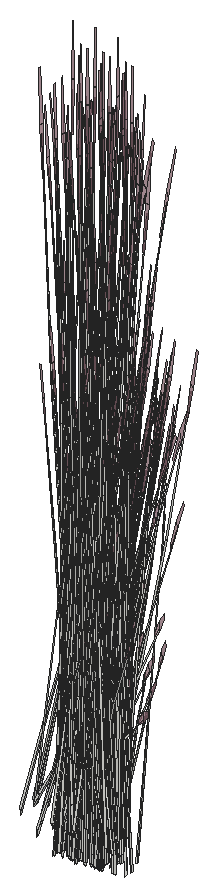
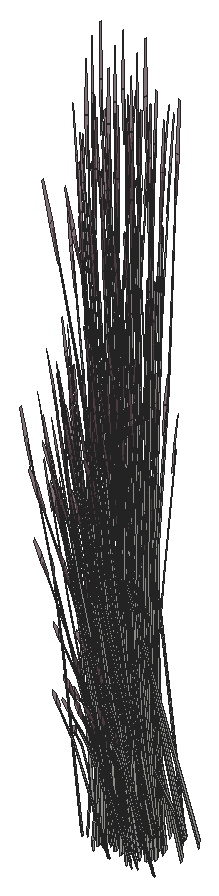
# SketchUp Ruby script. Lengths in inches.
U = 1.inch
M = Sketchup.active_model
def pt(a) = Geom::Point3d.new(a.map { |v| v * U })
def face(e, loops, mat)
  f = e.add_face(loops[0].map { |a| pt(a) })
  loops[1..].each { |l| e.add_face(l.map { |a| pt(a) }).erase! }
  f.material = f.back_material = mat if mat
  f
end
# faces: each face lists its corners as indices into pts; further lists are holes
def faces(e, pts, list, mat = nil) = list.each { |f| face(e, (f[0].is_a?(Array) ? f : [f]).map { |l| l.map { |i| pts[i] } }, mat) }
# xy, xz, yz: faces in a plane at the given z, y or x. An outline is a flat list of corners, or four numbers for a rectangle; further outlines are holes
def ring(l) = l.size == 4 ? [[l[0], l[1]], [l[2], l[1]], [l[2], l[3]], [l[0], l[3]]] : l.each_slice(2).to_a
def flat(e, list, mat, &to3) = list.each { |f| face(e, (f[0].is_a?(Array) ? f : [f]).map { |l| ring(l).map { |u, v| to3.(u, v) } }, mat) }
def xy(e, z, list, mat = nil) = flat(e, list, mat) { |x, y| [x, y, z] }
def xz(e, y, list, mat = nil) = flat(e, list, mat) { |x, z| [x, y, z] }
def yz(e, x, list, mat = nil) = flat(e, list, mat) { |y, z| [x, y, z] }
def lines(e, pts, list) = list.each { |a, b| e.add_line(pt(pts[a]), pt(pts[b])) }
# prism: a flat outline (further loops are holes) pulled along v
def prism(e, loops, v, mat = nil)
  f = face(e, loops, mat); d = Geom::Vector3d.new(v.map { |x| x * U })
  f.pushpull(f.normal.samedirection?(d) ? d.length : -d.length)
end
def box(e, o, s, mat = nil) = prism(e, [[o, [o[0] + s[0], o[1], o[2]], [o[0] + s[0], o[1] + s[1], o[2]], [o[0], o[1] + s[1], o[2]]]], [0, 0, s[2]], mat)
def at(x, y, z, deg = 0) = Geom::Transformation.translation(pt([x, y, z])) * Geom::Transformation.rotation(ORIGIN, Z_AXIS, deg.degrees)
def axes(o, x, y, z) = Geom::Transformation.new([*x, 0, *y, 0, *z, 0, *pt(o).to_a, 1])
def part(name) = M.definitions.add(name)
# library, detail: a bought-in or finely detailed component or shape, given as its bounding box
def library(name, o, s) = part(name).tap { |d| box(d.entities, o, s) }
def detail(e, o, s) = box(e.add_group.entities, o, s)
def put(e, d, t, mat = nil) = e.add_instance(d, t).tap { |i| i.material = mat if mat }
def group(e, t, mat = nil) = e.add_group.tap { |g| g.transformation = t; g.material = mat if mat }.entities
root = M.entities
M.materials.add("LightPink_Translucent").color = [144, 107, 117]
M.materials["LightPink_Translucent"].alpha = 0.75
c1 = part("blade")
p = [[2.15,0.21,22],[0,0.17,0],[0.09,0.45,0],[2.18,0.31,22],[2.29,0.31,22],[0.38,0.45,0],
  [2.48,0.24,33],[2.49,0.24,33],[2.48,0.22,33]]
faces(c1.entities,p,[[0,1,2,3],[4,5,2,3],[6,3,4,7],[8,0,3,6]])
c2 = part("seeds")
p = [[0.3,-0.1,1.38],[-0.01,-0.03,1.59],[-0.01,-0.03,0.03],[0.14,-0.07,-0.07],[0.29,-0.03,3],[0.15,0.01,3.11]]
faces(c2.entities,p,[[0,1,2,3],[1,0,4,5]],"LightPink_Translucent")
c3 = part("blade with seeds")
put(c3.entities,c1,at(0,0,0))
put(c3.entities,c2,axes([2.4,0.25,30.99],[1.5799,-0.05474,1.17369],[-0.12525,1.92788,0.29478],[-0.07173,-0.02425,1.56792]))
put(root,c3,axes([345.1,355.31,620.47],[-0.2773,-0.3397,0.17642],[0.27945,-0.32949,0.35086],[-0.03063,0.06937,1.60407]))
put(root,c3,axes([340.66,355.59,620.77],[-0.21807,0.07699,1.1486],[0.10265,-0.31819,0.84392],[0.11568,0.02177,0.25299]))
put(root,c3,axes([345.92,356.45,620.2],[-0.35581,-0.20937,0],[0.17124,-0.43505,0],[0,0,1.62707]))
put(root,c3,axes([346.22,355.89,620.46],[-0.34464,-0.37536,-0.25192],[0.29,-0.42149,0.5513],[-0.0928,0.04391,1.68216]))
put(root,c3,axes([347.07,354.85,622.72],[-0.05763,0.06055,1.74944],[0.0049,0.44239,-0.27667],[-0.13211,0.05753,0.14031]))
put(root,c3,axes([345.3125,356.61,620.48],[0.33032,0.23318,0.49651],[-0.19744,0.41812,0],[-0.07523,-0.05311,1.57504]))
put(root,c3,axes([347.45,354.79,622.68],[-0.09562,0.42421,-0.51099],[-0.32782,-0.1454,-0.3958],[-0.13199,0.0389,0.97773]))
put(root,c3,axes([347.4375,354.42,623.03],[0.17758,0.42229,-0.1216],[-0.31518,0.20752,-0.67495],[-0.13282,0.05572,1.02557]))
put(root,c3,axes([343.88,356.54,620.2],[-0.35581,-0.20937,0],[0.17124,-0.43505,0],[0,0,1.62707]))
put(root,c3,axes([344.18,355.98,620.46],[-0.34464,-0.37536,-0.25192],[0.29,-0.42149,0.5513],[-0.0928,0.04391,1.68216]))
put(root,c3,axes([348.1875,356.6,620.375],[-0.22066,0.46731,0],[-0.36918,-0.26061,-0.51607],[-0.08408,-0.05936,1.63711]))
put(root,c3,axes([343.27,356.7,620.48],[0.33032,0.23318,0.49651],[-0.19744,0.41812,0],[-0.07523,-0.05311,1.57504]))
put(root,c3,axes([342.5625,354.98,620.72],[0.17124,-0.42022,0.44739],[0.35581,0.20224,-0.21531],[0,0.09687,1.43643]))
put(root,c3,axes([346.48,354.99,620.72],[0.17124,-0.42022,0.44739],[0.35581,0.20224,-0.21531],[0,0.09687,1.43643]))
put(root,c3,axes([344.24,356.86,622.71],[-0.03191,-0.04083,1.77383],[0.06981,-0.43764,-0.16761],[0.12571,-0.02796,0.31391]))
put(root,c3,axes([344.43,355.08,620.72],[0.17124,-0.42022,0.44739],[0.35581,0.20224,-0.21531],[0,0.09687,1.43643]))
put(root,c3,axes([340.5625,356.94,622.71],[-0.03191,-0.04083,1.77383],[0.06981,-0.43764,-0.16761],[0.12571,-0.02796,0.31391]))
put(root,c3,axes([342.5,355.22,620.29],[0,0.53934,-0.05637],[-0.44133,0,0],[0,0.01695,1.79368]))
put(root,c3,axes([346.41,355.23,620.29],[0,0.53934,-0.05637],[-0.44133,0,0],[0,0.01695,1.79368]))
put(root,c3,axes([344.39,355.04,622.68],[-0.09562,0.42421,-0.51099],[-0.32782,-0.1454,-0.3958],[-0.13199,0.0389,0.97773]))
put(root,c3,axes([344.37,354.68,623.03],[0.17758,0.42229,-0.1216],[-0.31518,0.20752,-0.67495],[-0.13282,0.05572,1.02557]))
put(root,c3,axes([342.53,354.84,620.21],[0.21202,0.39143,-0.44739],[-0.32115,0.27564,0.21531],[0.06861,0.04843,1.43643]))
put(root,c3,axes([343.96,356.5,621.93],[-0.06755,-0.39203,-0.03492],[0.31928,-0.09013,-0.15832],[0.06667,0.02485,0.52218]))
put(root,c3,axes([345.12,356.85,620.375],[-0.22066,0.46731,0],[-0.36918,-0.26061,-0.51607],[-0.08408,-0.05936,1.63711]))
put(root,c3,axes([343.13,356.49,623.03],[0.0189,-0.47427,-0.1216],[0.35781,0.01296,-0.67495],[0.13781,0.03295,1.02557]))
put(root,c3,axes([344.37,355.32,620.29],[0,0.53934,-0.05637],[-0.44133,0,0],[0,0.01695,1.79368]))
put(root,c3,axes([344.4,354.94,620.21],[0.21202,0.39143,-0.44739],[-0.32115,0.27564,0.21531],[0.06861,0.04843,1.43643]))
put(root,c3,axes([343.46,355.22,620.48],[0,-0.46636,0.49651],[0.39487,0,0],[0,0.10622,1.57504]))
put(root,c3,axes([339.46,356.5625,623.03],[0.0189,-0.47427,-0.1216],[0.35781,0.01296,-0.67495],[0.13781,0.03295,1.02557]))
put(root,c3,axes([342.47,355.57,620.72],[0.38326,-0.02879,0.44739],[0.03466,0.47788,-0.21531],[-0.06861,0.04843,1.43643]))
put(root,c3,axes([346.39,355.58,620.72],[0.38326,-0.02879,0.44739],[0.03466,0.47788,-0.21531],[-0.06861,0.04843,1.43643]))
put(root,c3,axes([342.71,355.08,620.62],[0.32884,-0.136,0.1448],[0.11516,0.38837,-0.41347],[0,0.08547,1.26744]))
put(root,c3,axes([345.33,355.32,620.48],[0,-0.46636,0.49651],[0.39487,0,0],[0,0.10622,1.57504]))
put(root,c3,axes([343.08,356.3,623.05],[-0.20082,-0.29199,0.35414],[0.2293,-0.2764,-0.4572],[0.1165,0.04206,0.87481]))
put(root,c3,axes([344.34,355.67,620.72],[0.38326,-0.02879,0.44739],[0.03466,0.47788,-0.21531],[-0.06861,0.04843,1.43643]))
put(root,c3,axes([344.58,355.18,620.62],[0.32884,-0.136,0.1448],[0.11516,0.38837,-0.41347],[0,0.08547,1.26744]))
put(root,c3,axes([346.05,355.81,620.21],[-0.38326,0.02879,-0.44739],[-0.03466,-0.47788,0.21531],[-0.06861,0.04843,1.43643]))
put(root,c3,axes([344,355.9,620.21],[-0.38326,0.02879,-0.44739],[-0.03466,-0.47788,0.21531],[-0.06861,0.04843,1.43643]))
put(root,c3,axes([340.25,356.1,620.59],[-0.085,-0.1147,1.43002],[0.1106,-0.37943,-0.30754],[0.17198,0.0514,0.61141]))
put(root,c3,axes([347.4,355.61,622.73],[-0.08753,-0.42921,0.48003],[0.34336,-0.07449,0.3958],[-0.1012,0.10094,0.9933]))
put(root,c3,axes([347.33,355.52,622.73],[-0.2423,-0.19613,0.0643],[0.14107,-0.2793,0.50621],[-0.07768,0.0903,0.77189]))
put(root,c3,axes([347.44,355.01,621.875],[0.12246,-0.09864,1.71376],[0.1031,0.45582,0.13857],[-0.19225,0.10302,0.73262]))
put(root,c3,axes([342.41,356.44,620.2],[0.35581,0.20937,0],[-0.17124,0.43505,0],[0,0,1.74954]))
put(root,c3,axes([346.33,356.45,620.2],[0.35581,0.20937,0],[-0.17124,0.43505,0],[0,0,1.74954]))
put(root,c3,axes([344.28,356.54,620.2],[0.35581,0.20937,0],[-0.17124,0.43505,0],[0,0,1.74954]))
put(root,c3,axes([343.44,356.2,622.72],[0.07571,-0.00789,1.74944],[0.20767,-0.36231,-0.27667],[0.13467,0.04783,0.14031]))
put(root,c3,axes([346.47,356.92,620.19],[-0.21791,-0.46895,-0.05142],[0.36918,-0.26061,0.51607],[-0.09097,0.04465,1.6363]))
put(root,c3,axes([342.48,355.77,620.62],[0.26075,0.2802,0.1448],[-0.2175,0.31612,-0.41347],[-0.06054,0.04274,1.26744]))
put(root,c3,axes([346.39,355.78,620.62],[0.26075,0.2802,0.1448],[-0.2175,0.31612,-0.41347],[-0.06054,0.04274,1.26744]))
put(root,c3,axes([344.33,355.86,622.73],[-0.08753,-0.42921,0.48003],[0.34336,-0.07449,0.3958],[-0.1012,0.10094,0.9933]))
put(root,c3,axes([339.77,356.28,622.72],[0.07571,-0.00789,1.74944],[0.20767,-0.36231,-0.27667],[0.13467,0.04783,0.14031]))
put(root,c3,axes([344.27,355.77,622.73],[-0.2423,-0.19613,0.0643],[0.14107,-0.2793,0.50621],[-0.07768,0.0903,0.77189]))
put(root,c3,axes([344.43,357.01,620.19],[-0.21791,-0.46895,-0.05142],[0.36918,-0.26061,0.51607],[-0.09097,0.04465,1.6363]))
put(root,c3,axes([344.35,355.875,620.62],[0.26075,0.2802,0.1448],[-0.2175,0.31612,-0.41347],[-0.06054,0.04274,1.26744]))
put(root,c3,axes([347.06,355.78,620.59],[0.12266,0.03828,1.43002],[0.07906,0.39104,-0.30754],[-0.16661,0.0732,0.61141]))
put(root,c3,axes([343.15,356.26,622.98],[0.35281,0.01123,-0.71045],[-0.0237,0.47284,0.08574],[0.14947,0.0499,1.00501]))
put(root,c3,axes([347.61,355.46,623.05],[0.30722,-0.06665,0.35414],[0.08112,0.381,-0.4572],[-0.08804,0.10234,0.87481]))
put(root,c3,axes([342.75,356.64,620.48],[0.33032,-0.23318,0.49651],[0.19744,0.41812,0],[-0.07523,0.05311,1.57504]))
put(root,c3,axes([339.47,356.34,622.98],[0.35281,0.01123,-0.71045],[-0.0237,0.47284,0.08574],[0.14947,0.0499,1.00501]))
put(root,c3,axes([346.43,355.29,622.71],[0.04504,0.01251,1.77383],[0.13934,0.41205,-0.16761],[-0.0922,0.10815,0.31391]))
put(root,c3,axes([346.67,356.65,620.48],[0.33032,-0.23318,0.49651],[0.19744,0.41812,0],[-0.07523,0.05311,1.57504]))
put(root,c3,axes([342.28,356.27,620.29],[0.15345,0.53576,-0.06012],[-0.43845,0.18773,0],[0.00536,0.01871,1.72173]))
put(root,c3,axes([346.2,356.28,620.29],[0.15345,0.53576,-0.06012],[-0.43845,0.18773,0],[0.00536,0.01871,1.72173]))
put(root,c3,axes([344.625,356.74,620.48],[0.33032,-0.23318,0.49651],[0.19744,0.41812,0],[-0.07523,0.05311,1.57504]))
put(root,c3,axes([346.8,356.6,620.77],[0.14709,-0.21136,1.1486],[0.05804,0.3346,0.84392],[-0.1063,0.05991,0.25299]))
put(root,c3,axes([346.37,356.86,620.03],[-0.32928,-0.11539,-0.30978],[0.08291,-0.40636,0.30978],[-0.06638,0.04686,1.38974]))
put(root,c3,axes([344.16,356.37,620.29],[0.15345,0.53576,-0.06012],[-0.43845,0.18773,0],[0.00536,0.01871,1.72173]))
put(root,c3,axes([344.33,356.95,620.03],[-0.32928,-0.11539,-0.30978],[0.08291,-0.40636,0.30978],[-0.06638,0.04686,1.38974]))
put(root,c3,axes([344.54,355.71,623.05],[0.30722,-0.06665,0.35414],[0.08112,0.381,-0.4572],[-0.08804,0.10234,0.87481]))
put(root,c3,axes([343.73,355.3,620.375],[0.44133,0,0],[0,0.52122,-0.51607],[0,0.11871,1.63711]))
put(root,c3,axes([347.36,355.6875,622.53],[-0.30722,0.06665,-0.35414],[-0.08112,-0.381,0.4572],[-0.08804,0.10234,0.87481]))
put(root,c3,axes([343.55,355.57,620.2],[-0.44111,-0.00373,-0.04976],[0,-0.52122,0.49943],[-0.01386,0.11865,1.58352]))
put(root,c3,axes([343.36,355.54,622.71],[0.04504,0.01251,1.77383],[0.13934,0.41205,-0.16761],[-0.0922,0.10815,0.31391]))
put(root,c3,axes([347.47,355.58,620.2],[-0.44111,-0.00373,-0.04976],[0,-0.52122,0.49943],[-0.01386,0.11865,1.58352]))
put(root,c3,axes([342.6,355.11,620.67],[0.39748,0.22252,-0.29095],[-0.19139,0.46966,-0.50002],[0.01249,0.11531,1.59708]))
put(root,c3,axes([345.6,355.4,620.375],[0.44133,0,0],[0,0.52122,-0.51607],[0,0.11871,1.63711]))
put(root,c3,axes([343.36,356.45,622.53],[0.20082,0.29199,-0.35414],[-0.2293,0.2764,0.4572],[0.1165,0.04206,0.87481]))
put(root,c3,axes([343.46,355.64,620.03],[-0.24637,0.29097,-0.30978],[-0.24637,-0.29097,0.30978],[0,0.09372,1.38974]))
put(root,c3,axes([345.42,355.67,620.2],[-0.44111,-0.00373,-0.04976],[0,-0.52122,0.49943],[-0.01386,0.11865,1.58352]))
put(root,c3,axes([343.74,356.85,620.77],[0.14709,-0.21136,1.1486],[0.05804,0.3346,0.84392],[-0.1063,0.05991,0.25299]))
put(root,c3,axes([344.47,355.21,620.67],[0.39748,0.22252,-0.29095],[-0.19139,0.46966,-0.50002],[0.01249,0.11531,1.59708]))
put(root,c3,axes([346.3125,355.68,620.67],[0.04113,0.53214,-0.29095],[-0.42835,0.03218,-0.50002],[-0.07543,0.07088,1.59708]))
put(root,c3,axes([343.26,356.5625,622.73],[-0.01777,0.35463,0.0643],[-0.26836,-0.00972,0.50621],[0.1028,0.03711,0.77189]))
put(root,c3,axes([339.69,356.53,622.53],[0.20082,0.29199,-0.35414],[-0.2293,0.2764,0.4572],[0.1165,0.04206,0.87481]))
put(root,c3,axes([342.55,355.46,620.21],[-0.17124,0.42022,-0.44739],[-0.35581,-0.20224,0.21531],[0,0.09687,1.43643]))
put(root,c3,axes([346.47,355.47,620.21],[-0.17124,0.42022,-0.44739],[-0.35581,-0.20224,0.21531],[0,0.09687,1.43643]))
put(root,c3,axes([345.33,355.74,620.03],[-0.24637,0.29097,-0.30978],[-0.24637,-0.29097,0.30978],[0,0.09372,1.38974]))
put(root,c3,axes([344.29,355.9375,622.53],[-0.30722,0.06665,-0.35414],[-0.08112,-0.381,0.4572],[-0.08804,0.10234,0.87481]))
put(root,c3,axes([344.27,355.77,620.67],[0.04113,0.53214,-0.29095],[-0.42835,0.03218,-0.50002],[-0.07543,0.07088,1.59708]))
put(root,c3,axes([343.29,356.45,622.73],[-0.26024,0.30729,0.48003],[-0.22444,-0.32634,0.3958],[0.1221,0.05668,0.9933]))
put(root,c3,axes([346.91,356.55,623.65],[0.31145,0.12449,-0.06488],[-0.0958,0.38314,-0.29416],[-0.05094,0.05817,0.97024]))
put(root,c3,axes([344.43,355.5625,620.21],[-0.17124,0.42022,-0.44739],[-0.35581,-0.20224,0.21531],[0,0.09687,1.43643]))
put(root,c3,axes([343.85,356.8,623.65],[0.31145,0.12449,-0.06488],[-0.0958,0.38314,-0.29416],[-0.05094,0.05817,0.97024]))
put(root,c3,axes([346.06,356.09,620.06],[-0.23773,0.35053,-0.62353],[-0.29532,-0.31785,-0.16365],[-0.09526,0.08744,1.37633]))
put(root,c3,axes([342.46,356.81,623.05],[-0.05451,-0.37564,0.35414],[0.31161,-0.09919,-0.4572],[0.0837,0.10765,0.87481]))
put(root,c3,axes([344.01,356.18,620.06],[-0.23773,0.35053,-0.62353],[-0.29532,-0.31785,-0.16365],[-0.09526,0.08744,1.37633]))
put(root,c3,axes([347.45,355.43,623.03],[0.32648,0.25715,-0.1216],[-0.18809,0.3724,-0.67495],[-0.09224,0.12945,1.02557]))
put(root,c3,axes([342.5625,356.67,620.33],[0.44186,0.15158,0.30756],[-0.11054,0.54181,-0.36492],[-0.07313,0.06781,1.64885]))
put(root,c3,axes([346.48,356.68,620.33],[0.44186,0.15158,0.30756],[-0.11054,0.54181,-0.36492],[-0.07313,0.06781,1.64885]))
put(root,c3,axes([343.63,355.65,620.02],[0,0.46636,-0.49651],[-0.39487,0,0],[0,0.10622,1.57504]))
put(root,c3,axes([346.45,357.04,620.02],[-0.33032,0.23318,-0.49651],[-0.19744,-0.41812,0],[-0.07523,0.05311,1.57504]))
put(root,c3,axes([342.64,355.7,621.875],[-0.1311,-0.08035,1.71376],[0.27131,-0.33708,0.13857],[0.16909,0.15206,0.73262]))
put(root,c3,axes([344.33,356.91,623.05],[-0.05451,-0.37564,0.35414],[0.31161,-0.09919,-0.4572],[0.0837,0.10765,0.87481]))
put(root,c3,axes([344.43,356.77,620.33],[0.44186,0.15158,0.30756],[-0.11054,0.54181,-0.36492],[-0.07313,0.06781,1.64885]))
put(root,c3,axes([342.67,354.65,622.47],[-0.30498,-0.24231,1.38283],[0.32203,-0.37727,0.59665],[0.0984,0.22736,1.33663]))
put(root,c3,axes([344.4,357.13,620.02],[-0.33032,0.23318,-0.49651],[-0.19744,-0.41812,0],[-0.07523,0.05311,1.57504]))
put(root,c3,axes([345.5,355.75,620.02],[0,0.46636,-0.49651],[-0.39487,0,0],[0,0.10622,1.57504]))
put(root,c3,axes([338.96,355.78,621.875],[-0.1311,-0.08035,1.71376],[0.27131,-0.33708,0.13857],[0.16909,0.15206,0.73262]))
put(root,c3,axes([347.89,355.3125,621.875],[0.08815,-0.14329,1.71376],[0.22258,0.38678,0.13857],[-0.15267,0.17614,0.73262]))
put(root,c3,axes([347.61,355.73,622.68],[0.09067,0.42583,-0.51099],[-0.34336,0.07449,-0.3958],[-0.0984,0.11438,0.97773]))
put(root,c3,axes([344.54,354.75,622.47],[-0.30498,-0.24231,1.38283],[0.32203,-0.37727,0.59665],[0.0984,0.22736,1.33663]))
put(root,c3,axes([344.38,355.68,623.03],[0.32648,0.25715,-0.1216],[-0.18809,0.3724,-0.67495],[-0.09224,0.12945,1.02557]))
put(root,c3,axes([343.13,356.62,620.77],[-0.19872,-0.13409,1.1486],[0.2566,-0.13625,0.84392],[0.06921,0.11541,0.25299]))
put(root,c3,axes([342.43,357,623.03],[0.21031,-0.39918,-0.1216],[0.30457,0.22997,-0.67495],[0.10587,0.11278,1.02557]))
put(root,c3,axes([345,356.72,620.77],[-0.19872,-0.13409,1.1486],[0.2566,-0.13625,0.84392],[0.06921,0.11541,0.25299]))
put(root,c3,axes([344.3,357.1,623.03],[0.21031,-0.39918,-0.1216],[0.30457,0.22997,-0.67495],[0.10587,0.11278,1.02557]))
put(root,c3,axes([344.82,355.5625,621.875],[0.08815,-0.14329,1.71376],[0.22258,0.38678,0.13857],[-0.15267,0.17614,0.73262]))
put(root,c3,axes([347.19,356.82,619.49],[0.04734,0.04659,1.76342],[0.08027,0.4317,-0.26939],[-0.10492,0.09206,0.30037]))
put(root,c3,axes([347.9,356.47,622.73],[-0.25132,-0.3182,0.48003],[0.2669,-0.27442,0.3958],[-0.04636,0.14929,0.9933]))
put(root,c3,axes([344.55,355.98,622.68],[0.09067,0.42583,-0.51099],[-0.34336,0.07449,-0.3958],[-0.0984,0.11438,0.97773]))
put(root,c3,axes([344.96,356.47,623.05],[0.23881,-0.24554,0.35414],[0.22606,0.28036,-0.4572],[-0.0344,0.14245,0.87481]))
put(root,c3,axes([346.75,356.97,620.375],[0.22066,0.46731,0],[-0.36918,0.26061,-0.51607],[-0.08408,0.05936,1.63711]))
put(root,c3,axes([342.15,357.33,622.71],[0.00104,-0.05646,1.77383],[0.30246,-0.2491,-0.16761],[0.10506,0.08891,0.31391]))
put(root,c3,axes([343.18,357.12,619.49],[0.02571,-0.06733,1.76342],[0.32373,-0.19829,-0.26939],[0.09815,0.10263,0.30037]))
put(root,c3,axes([342.91,356.5625,623.05],[0.23881,-0.24554,0.35414],[0.22606,0.28036,-0.4572],[-0.0344,0.14245,0.87481]))
put(root,c3,axes([342.76,355.59,620.09],[0.12941,0.42699,-0.69212],[-0.37279,0.15378,-0.18165],[0.0143,0.14459,1.52773]))
put(root,c3,axes([346.56,355.12,620.84],[-0.00964,-0.43909,1.41272],[0.43635,0.11382,0.59816],[-0.1032,0.24027,1.3335]))
put(root,c3,axes([344.7,357.06,620.375],[0.22066,0.46731,0],[-0.36918,0.26061,-0.51607],[-0.08408,0.05936,1.63711]))
put(root,c3,axes([344.74,356.7,622.73],[-0.29004,-0.02173,0.0643],[0.00795,-0.32812,0.50621],[-0.03035,0.12569,0.77189]))
put(root,c3,axes([344.125,357.07,619.49],[0.04734,0.04659,1.76342],[0.08027,0.4317,-0.26939],[-0.10492,0.09206,0.30037]))
put(root,c3,axes([342.68,356.8,622.68],[0.34827,-0.11086,-0.51099],[0.06092,0.41983,-0.3958],[0.09354,0.12031,0.97773]))
put(root,c3,axes([344.03,357.43,622.71],[0.00104,-0.05646,1.77383],[0.30246,-0.2491,-0.16761],[0.10506,0.08891,0.31391]))
put(root,c3,axes([344.83,356.73,622.73],[-0.25132,-0.3182,0.48003],[0.2669,-0.27442,0.3958],[-0.04636,0.14929,0.9933]))
put(root,c3,axes([344.51,355.21,620.84],[-0.00964,-0.43909,1.41272],[0.43635,0.11382,0.59816],[-0.1032,0.24027,1.3335]))
put(root,c3,axes([344.63,355.6875,620.09],[0.12941,0.42699,-0.69212],[-0.37279,0.15378,-0.18165],[0.0143,0.14459,1.52773]))
put(root,c3,axes([342.7,356.79,622.73],[-0.29004,-0.02173,0.0643],[0.00795,-0.32812,0.50621],[-0.03035,0.12569,0.77189]))
put(root,c3,axes([341.71,356.87,623.05],[0.1064,-0.35863,0.35414],[0.31043,0.1046,-0.4572],[0.02846,0.14439,0.87481]))
put(root,c3,axes([345.63,356.875,623.05],[0.1064,-0.35863,0.35414],[0.31043,0.1046,-0.4572],[0.02846,0.14439,0.87481]))
put(root,c3,axes([342.79,356.82,622.73],[-0.25132,-0.3182,0.48003],[0.2669,-0.27442,0.3958],[-0.04636,0.14929,0.9933]))
put(root,c3,axes([344.55,356.9,622.68],[0.34827,-0.11086,-0.51099],[0.06092,0.41983,-0.3958],[0.09354,0.12031,0.97773]))
put(root,c3,axes([343.58,356.97,623.05],[0.1064,-0.35863,0.35414],[0.31043,0.1046,-0.4572],[0.02846,0.14439,0.87481]))
put(root,c3,axes([343.16,357.23,620.67],[-0.22633,-0.01463,1.0506],[0.14947,-0.31064,0.58006],[0.08941,0.11036,0.8241]))
put(root,c3,axes([345.03,357.33,620.67],[-0.22633,-0.01463,1.0506],[0.14947,-0.31064,0.58006],[0.08941,0.11036,0.8241]))
put(root,c3,axes([347.82,355.67,621.875],[0.06572,-0.16029,1.71376],[0.27569,0.33172,0.13857],[-0.12437,0.20675,0.73262]))
put(root,c3,axes([342.51,357.15,622.73],[-0.16041,0.29625,0.0643],[-0.22843,-0.17248,0.50621],[0.07385,0.09498,0.77189]))
put(root,c3,axes([342.13,358.15,623.65],[0.2439,-0.26754,-0.06488],[0.22348,0.29302,-0.29416],[0.01573,0.08303,0.97024]))
put(root,c3,axes([346.05,358.16,623.65],[0.2439,-0.26754,-0.06488],[0.22348,0.29302,-0.29416],[0.01573,0.08303,0.97024]))
put(root,c3,axes([344.38,357.25,622.73],[-0.16041,0.29625,0.0643],[-0.22843,-0.17248,0.50621],[0.07385,0.09498,0.77189]))
put(root,c3,axes([342.57,357.0625,622.73],[-0.35104,0.10702,0.48003],[-0.06092,-0.41983,0.3958],[0.08256,0.12373,0.9933]))
put(root,c3,axes([344,358.25,623.65],[0.2439,-0.26754,-0.06488],[0.22348,0.29302,-0.29416],[0.01573,0.08303,0.97024]))
put(root,c3,axes([347.08,356.5,622.72],[-0.00877,0.09229,1.74944],[0.24897,0.32105,-0.27667],[-0.06518,0.15182,0.14031]))
put(root,c3,axes([344.45,357.16,622.73],[-0.35104,0.10702,0.48003],[-0.06092,-0.41983,0.3958],[0.08256,0.12373,0.9933]))
put(root,c3,axes([344.76,355.92,621.875],[0.06572,-0.16029,1.71376],[0.27569,0.33172,0.13857],[-0.12437,0.20675,0.73262]))
put(root,c3,axes([342.42,356.48,620.59],[0.00623,-0.15459,1.43002],[0.29764,-0.17268,-0.30754],[0.09188,0.18503,0.61141]))
put(root,c3,axes([341.62,357.19,622.73],[-0.26007,0.1585,0.0643],[-0.12729,-0.28902,0.50621],[0.02512,0.1274,0.77189]))
put(root,c3,axes([344.29,356.58,620.59],[0.00623,-0.15459,1.43002],[0.29764,-0.17268,-0.30754],[0.09188,0.18503,0.61141]))
put(root,c3,axes([345.53,357.2,622.73],[-0.26007,0.1585,0.0643],[-0.12729,-0.28902,0.50621],[0.02512,0.1274,0.77189]))
put(root,c3,axes([344.83,356.82,622.53],[-0.23881,0.24554,-0.35414],[-0.22606,-0.28036,0.4572],[-0.0344,0.14245,0.87481]))
put(root,c3,axes([344.01,356.75,622.72],[-0.00877,0.09229,1.74944],[0.24897,0.32105,-0.27667],[-0.06518,0.15182,0.14031]))
put(root,c3,axes([344.81,356.54,623.4],[0.3879,0.02311,-0.13498],[-0.0106,0.43749,-0.74919],[-0.02694,0.1685,1.13838]))
put(root,c3,axes([341.61,357.02,623.03],[0.34538,-0.21713,-0.1216],[0.16972,0.38536,-0.67495],[0.04557,0.16239,1.02557]))
put(root,c3,axes([341.71,357.16,623.0625],[-0.34777,-0.12192,0.53283],[0.11892,-0.40083,0.43934],[0.0209,0.15763,1.10256]))
put(root,c3,axes([345.625,357.17,623.0625],[-0.34777,-0.12192,0.53283],[0.11892,-0.40083,0.43934],[0.0209,0.15763,1.10256]))
put(root,c3,axes([343.49,357.29,622.73],[-0.26007,0.1585,0.0643],[-0.12729,-0.28902,0.50621],[0.02512,0.1274,0.77189]))
put(root,c3,axes([342.79,356.91,622.53],[-0.23881,0.24554,-0.35414],[-0.22606,-0.28036,0.4572],[-0.0344,0.14245,0.87481]))
put(root,c3,axes([342.76,356.63,623.4],[0.3879,0.02311,-0.13498],[-0.0106,0.43749,-0.74919],[-0.02694,0.1685,1.13838]))
put(root,c3,axes([344.99,357.77,620.77],[-0.00913,-0.2773,1.1486],[0.22824,0.19778,0.84392],[-0.04489,0.13217,0.25299]))
put(root,c3,axes([343.48,357.12,623.03],[0.34538,-0.21713,-0.1216],[0.16972,0.38536,-0.67495],[0.04557,0.16239,1.02557]))
put(root,c3,axes([343.58,357.26,623.0625],[-0.34777,-0.12192,0.53283],[0.11892,-0.40083,0.43934],[0.0209,0.15763,1.10256]))
put(root,c3,axes([342.94,357.86,620.77],[-0.00913,-0.2773,1.1486],[0.22824,0.19778,0.84392],[-0.04489,0.13217,0.25299]))
put(root,c3,axes([341.67,357.1,619.49],[0.05712,-0.02538,1.76342],[0.34359,0.13968,-0.26939],[0.01005,0.15742,0.30037]))
put(root,c3,axes([345.59,357.11,619.49],[0.05712,-0.02538,1.76342],[0.34359,0.13968,-0.26939],[0.01005,0.15742,0.30037]))
put(root,c3,axes([343.54,357.2,619.49],[0.05712,-0.02538,1.76342],[0.34359,0.13968,-0.26939],[0.01005,0.15742,0.30037]))
put(root,c3,axes([345.07,356.7,623],[0.25266,0.31335,-0.5672],[-0.2669,0.27442,-0.43934],[-0.03844,0.15921,1.08528]))
put(root,c3,axes([341.91,357,622.68],[0.34695,0.11691,-0.51099],[-0.11892,0.40083,-0.3958],[0.03181,0.16138,0.97773]))
put(root,c3,axes([344.8,357.18,620.82],[0.32063,-0.08258,0.06507],[0.07371,0.33271,-0.86304],[-0.02033,0.16842,0.7736]))
put(root,c3,axes([342.1,356.17,621.875],[-0.08068,-0.14973,1.71376],[0.3728,-0.12606,0.13857],[0.08426,0.23506,0.73262]))
put(root,c3,axes([343.03,356.79,623],[0.25266,0.31335,-0.5672],[-0.2669,0.27442,-0.43934],[-0.03844,0.15921,1.08528]))
put(root,c3,axes([342.75,357.27,620.82],[0.32063,-0.08258,0.06507],[0.07371,0.33271,-0.86304],[-0.02033,0.16842,0.7736]))
put(root,c3,axes([343.78,357.1,622.68],[0.34695,0.11691,-0.51099],[-0.11892,0.40083,-0.3958],[0.03181,0.16138,0.97773]))
put(root,c3,axes([343.97,356.27,621.875],[-0.08068,-0.14973,1.71376],[0.3728,-0.12606,0.13857],[0.08426,0.23506,0.73262]))
put(root,c3,axes([341.75,357.24,622.53],[-0.1064,0.35863,-0.35414],[-0.31043,-0.1046,0.4572],[0.02846,0.14439,0.87481]))
put(root,c3,axes([345.66,357.25,622.53],[-0.1064,0.35863,-0.35414],[-0.31043,-0.1046,0.4572],[0.02846,0.14439,0.87481]))
put(root,c3,axes([343.62,357.34,622.53],[-0.1064,0.35863,-0.35414],[-0.31043,-0.1046,0.4572],[0.02846,0.14439,0.87481]))
put(root,c3,axes([344.99,356.5625,623.34],[-0.00918,0.43138,-0.7886],[-0.38672,-0.02897,0.09517],[-0.04081,0.18275,1.11556]))
put(root,c3,axes([343.98,357.69,622.71],[0.04004,-0.02816,1.77383],[0.33095,0.18728,-0.16761],[-0.00778,0.15594,0.31391]))
put(root,c3,axes([342.95,356.65,623.34],[-0.00918,0.43138,-0.7886],[-0.38672,-0.02897,0.09517],[-0.04081,0.18275,1.11556]))
put(root,c3,axes([341.9375,357.78,622.71],[0.04004,-0.02816,1.77383],[0.33095,0.18728,-0.16761],[-0.00778,0.15594,0.31391]))
put(root,c3,axes([345.36,356.26,621.875],[-0.00864,-0.17899,1.71376],[0.37441,0.11874,0.13857],[-0.02316,0.25508,0.73262]))
put(root,c3,axes([347.78,357.28,620.59],[0.11138,-0.07357,1.43002],[0.27499,0.22183,-0.30754],[-0.08185,0.19194,0.61141]))
put(root,c3,axes([343.31,356.35,621.875],[-0.00864,-0.17899,1.71376],[0.37441,0.11874,0.13857],[-0.02316,0.25508,0.73262]))
put(root,c3,axes([341.78,356.92,622.98],[0.16845,0.3792,-0.71045],[-0.34676,0.21133,0.08574],[0.03939,0.18322,1.00501]))
put(root,c3,axes([345.69,356.93,622.98],[0.16845,0.3792,-0.71045],[-0.34676,0.21133,0.08574],[0.03939,0.18322,1.00501]))
put(root,c3,axes([343.65,357.02,622.98],[0.16845,0.3792,-0.71045],[-0.34676,0.21133,0.08574],[0.03939,0.18322,1.00501]))
put(root,c3,axes([344.72,357.53,620.59],[0.11138,-0.07357,1.43002],[0.27499,0.22183,-0.30754],[-0.08185,0.19194,0.61141]))
